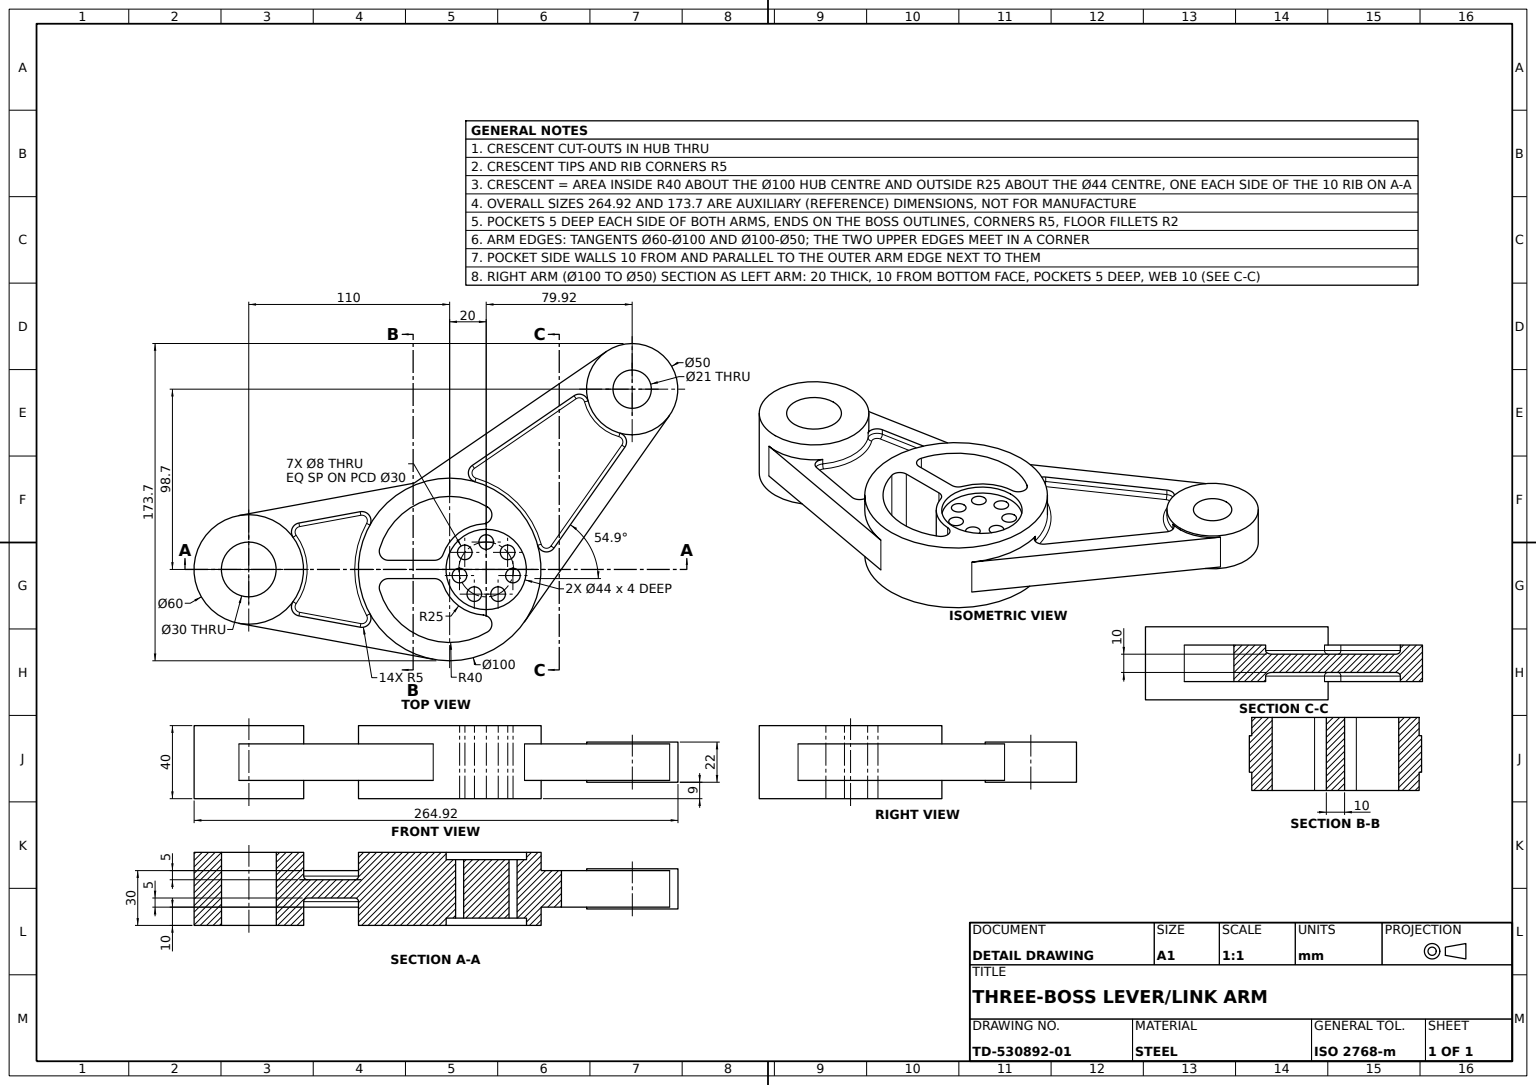
solid
v1 (-82.1770338609,5,-23.4495747344)
v2 (-82.5406702246,7,-25.4162390665)
e1 v1 v2 CIRCLE(AX(P(-82.1770338609,7,-23.4495747344),D(0.983332166,0,-0.1818181818),D(-0.1818181818,0,-0.983332166)),2)
v3 (-48.6283414749,5,-29.652730151)
e2 v3 v1 LINE
v4 (-48.9919778385,7,-31.619394483)
e3 v3 v4 CIRCLE(AX(P(-48.6283414749,7,-29.652730151),D(0.983332166,0,-0.1818181818),D(-0.1818181818,0,-0.983332166)),2)
e4 v2 v4 LINE
face CYL(AX(P(-6.9090909091,7,-37.3666223094),D(0.983332166,0,-0.1818181818),D(-0.1818181818,0,-0.983332166)),2) rev [-e1 -e2 e3 -e4]
v5 (57.1214748065,-7,-11.710555748)
v6 (57.1214748065,-10,-11.710555748)
e5 v5 v6 LINE
v7 (95.9321157128,-7,-66.9317168355)
e6 v5 v7 LINE
v8 (95.9321157128,-10,-66.9317168355)
e7 v7 v8 LINE
e8 v6 v8 LINE
face PLANE(AX(P(32.7258328837,10,23.0004317801),D(-0.8181458221,0,-0.5750107945),D(-0.5750107945,0,0.8181458221))) [-e5 e6 e7 -e8]
v9 (50.1381595672,-5,-13.7900310085)
v10 (14.4079942754,-5,-49.9640841101)
e9 v9 v10 CIRCLE(AX(P(0,-5,0),D(0,1,0),D(0,0,1)),52)
v11 (48.2097688146,-7,-13.2596452005)
e10 v9 v11 CIRCLE(AX(P(50.1381595672,-7,-13.7900310085),D(0.265192904,0,0.9641953763),D(0.9641953763,0,-0.265192904)),2)
v12 (13.8538406494,-7,-48.0423885674)
e11 v12 v11 CIRCLE(AX(P(0,-7,0),D(0,-1,0),D(0,0,1)),50)
e12 v10 v12 CIRCLE(AX(P(14.4079942754,-7,-49.9640841101),D(0.9608477713,0,0.277076813),D(0.277076813,0,-0.9608477713)),2)
face TORUS(AX(P(0,-7,0),D(0,1,0),D(0,0,1)),52,2) rev [-e9 e10 -e11 -e12]
v13 (-82.5406702246,10,-25.4162390665)
e13 v13 v2 LINE
v14 (-85.6842108418,10,-17.5710670597)
e14 v13 v14 CIRCLE(AX(P(-81.6315793155,10,-20.4995782363),D(0,1,0),D(0,0,1)),5)
v15 (-85.6842108418,7,-17.5710670597)
e15 v14 v15 LINE
e16 v15 v2 CIRCLE(AX(P(-81.6315793155,7,-20.4995782363),D(0,-1,0),D(0,0,1)),5)
face CYL(AX(P(-81.6315793155,10,-20.4995782363),D(0,-1,0),D(0,0,-1)),5) rev [-e13 e14 e15 e16]
v16 (-110,10,-30)
e17 v14 v16 CIRCLE(AX(P(-110,10,0),D(0,1,0),D(0,0,1)),30)
v17 (-110,20,-30)
e18 v17 v16 LINE
v18 (-110,20,30)
e19 v18 v17 CIRCLE(AX(P(-110,20,0),D(0,1,0),D(0,0,1)),30)
v19 (-110,10,30)
e20 v18 v19 LINE
v20 (-85.6842108418,10,17.5710670597)
e21 v19 v20 CIRCLE(AX(P(-110,10,0),D(0,1,0),D(0,0,1)),30)
v21 (-85.6842108418,7,17.5710670597)
e22 v20 v21 LINE
e23 v21 v15 CIRCLE(AX(P(-110,7,0),D(0,1,0),D(0,0,1)),30)
face CYL(AX(P(-110,20,0),D(0,-1,0),D(0,0,-1)),30) [e17 -e18 -e19 e20 e21 e22 e23 -e15]
v22 (5.3760813173,16,-0.6621859907)
v23 (5.3760813173,16,7.3378140093)
e24 v22 v23 CIRCLE(AX(P(5.3760813173,16,3.3378140093),D(0,1,0),D(0,0,1)),4)
v24 (5.3760813173,-16,7.3378140093)
e25 v23 v24 LINE
v25 (5.3760813173,-16,-0.6621859907)
e26 v25 v24 CIRCLE(AX(P(5.3760813173,-16,3.3378140093),D(0,1,0),D(0,0,1)),4)
e27 v22 v25 LINE
face CYL(AX(P(5.3760813173,16,3.3378140093),D(0,-1,0),D(0,0,-1)),4) rev [e24 e25 -e26 -e27]
v26 (20,-16,-19)
v27 (20,-16,-11)
e28 v26 v27 CIRCLE(AX(P(20,-16,-15),D(0,1,0),D(0,0,1)),4)
v28 (20,16,-19)
e29 v28 v26 LINE
v29 (20,16,-11)
e30 v28 v29 CIRCLE(AX(P(20,16,-15),D(0,1,0),D(0,0,1)),4)
e31 v29 v27 LINE
face CYL(AX(P(20,16,-15),D(0,-1,0),D(0,0,-1)),4) rev [-e28 -e29 e30 e31]
v30 (93.1884371125,10,-74.6218985242)
v31 (95.9321157128,10,-66.9317168355)
e32 v30 v31 CIRCLE(AX(P(91.8413866024,10,-69.806770808),D(0,-1,0),D(0,0,1)),5)
v32 (93.1884371125,7,-74.6218985242)
e33 v30 v32 LINE
v33 (95.9321157128,7,-66.9317168355)
e34 v32 v33 CIRCLE(AX(P(91.8413866024,7,-69.806770808),D(0,-1,0),D(0,0,1)),5)
e35 v31 v33 LINE
face CYL(AX(P(91.8413866024,10,-69.806770808),D(0,-1,0),D(0,0,-1)),5) rev [-e32 e33 e34 -e35]
v34 (-110,-20,15)
v35 (-110,-20,-15)
e36 v34 v35 CIRCLE(AX(P(-110,-20,0),D(0,1,0),D(0,0,1)),15)
v36 (-110,20,15)
e37 v36 v34 LINE
v37 (-110,20,-15)
e38 v36 v37 CIRCLE(AX(P(-110,20,0),D(0,1,0),D(0,0,1)),15)
e39 v37 v35 LINE
face CYL(AX(P(-110,20,0),D(0,-1,0),D(0,0,-1)),15) rev [-e36 -e37 e38 e39]
v38 (-110,-20,30)
v39 (-110,-20,-30)
e40 v38 v39 CIRCLE(AX(P(-110,-20,0),D(0,1,0),D(0,0,1)),30)
e41 v39 v38 CIRCLE(AX(P(-110,-20,0),D(0,1,0),D(0,0,1)),30)
e42 v35 v34 CIRCLE(AX(P(-110,-20,0),D(0,1,0),D(0,0,1)),15)
face PLANE(AX(P(-110,-20,0),D(0,1,0),D(0,0,1))) rev [-e40 -e41] [e36 e42]
v40 (69.2407418314,-5,-93.4480883396)
v41 (73.8341748162,-5,-91.7450400685)
e43 v40 v41 CIRCLE(AX(P(70.9353398332,-5,-90.9725403978),D(0,-1,0),D(0,0,1)),3)
v42 (68.1110098301,-7,-95.0984536341)
e44 v42 v40 CIRCLE(AX(P(69.2407418314,-7,-93.4480883396),D(0.8251826473,0,-0.5648660006),D(-0.5648660006,0,-0.8251826473)),2)
v43 (70.9353398332,-7,-95.9725403978)
e45 v43 v42 CIRCLE(AX(P(70.9353398332,-7,-90.9725403978),D(0,1,0),D(0,0,1)),5)
v44 (75.7667314716,-7,-92.260039849)
e46 v44 v43 CIRCLE(AX(P(70.9353398332,-7,-90.9725403978),D(0,1,0),D(0,0,1)),5)
e47 v44 v41 CIRCLE(AX(P(73.8341748162,-7,-91.7450400685),D(0.2574998902,0,0.9662783277),D(0.9662783277,0,-0.2574998902)),2)
face TORUS(AX(P(70.9353398332,-7,-90.9725403978),D(0,1,0),D(0,0,1)),3,2) rev [-e43 -e44 -e45 -e46 e47]
v45 (-38.3325939,-20,11.4285714286)
v46 (20.7142857143,-20,34.2186844772)
e48 v45 v46 CIRCLE(AX(P(0,-20,0),D(0,1,0),D(0,0,1)),40)
v47 (18.4375,-20,24.9511240979)
e49 v46 v47 CIRCLE(AX(P(18.125,-20,29.9413489175),D(0,1,0),D(0,0,-1)),5)
v48 (-3.5702260396,-20,8.3333333333)
e50 v47 v48 CIRCLE(AX(P(20,-20,0),D(0,-1,0),D(0,0,1)),25)
v49 (-8.2842712475,-20,5)
e51 v48 v49 CIRCLE(AX(P(-8.2842712475,-20,10),D(0,1,0),D(0,0,-1)),5)
v50 (-33.5410196625,-20,5)
e52 v49 v50 LINE
e53 v50 v45 CIRCLE(AX(P(-33.5410196625,-20,10),D(0,1,0),D(0,0,1)),5)
v51 (20,-20,22)
v52 (20,-20,-22)
e54 v51 v52 CIRCLE(AX(P(20,-20,0),D(0,1,0),D(0,0,1)),22)
e55 v52 v51 CIRCLE(AX(P(20,-20,0),D(0,1,0),D(0,0,1)),22)
v53 (20.7142857143,-20,-34.2186844772)
v54 (0,-20,-40)
e56 v53 v54 CIRCLE(AX(P(0,-20,0),D(0,1,0),D(0,0,1)),40)
v55 (-38.3325939,-20,-11.4285714286)
e57 v54 v55 CIRCLE(AX(P(0,-20,0),D(0,1,0),D(0,0,1)),40)
v56 (-33.5410196625,-20,-5)
e58 v55 v56 CIRCLE(AX(P(-33.5410196625,-20,-10),D(0,1,0),D(0,0,-1)),5)
v57 (-8.2842712475,-20,-5)
e59 v56 v57 LINE
v58 (-3.5702260396,-20,-8.3333333333)
e60 v57 v58 CIRCLE(AX(P(-8.2842712475,-20,-10),D(0,1,0),D(0,0,1)),5)
v59 (18.4375,-20,-24.9511240979)
e61 v58 v59 CIRCLE(AX(P(20,-20,0),D(0,-1,0),D(0,0,1)),25)
e62 v59 v53 CIRCLE(AX(P(18.125,-20,-29.9413489175),D(0,1,0),D(0,0,-1)),5)
v60 (0,-20,-50)
v61 (0,-20,50)
e63 v60 v61 CIRCLE(AX(P(0,-20,0),D(0,1,0),D(0,0,1)),50)
e64 v61 v60 CIRCLE(AX(P(0,-20,0),D(0,1,0),D(0,0,1)),50)
face PLANE(AX(P(0,-20,0),D(0,1,0),D(0,0,1))) rev [e48 e49 e50 e51 e52 e53] [e54 e55] [e56 e57 e58 e59 e60 e61 e62] [-e63 -e64]
v62 (50.1381595672,5,-13.7900310085)
v63 (53.0307456961,5,-11.5856097205)
e65 v62 v63 CIRCLE(AX(P(53.0307456961,5,-14.5856097205),D(0,1,0),D(0,0,1)),3)
v64 (55.4851831623,5,-12.860577337)
e66 v63 v64 CIRCLE(AX(P(53.0307456961,5,-14.5856097205),D(0,1,0),D(0,0,1)),3)
v65 (94.2958240686,5,-68.0817384245)
e67 v64 v65 LINE
v66 (92.6496169085,5,-72.6958474377)
e68 v65 v66 CIRCLE(AX(P(91.8413866024,5,-69.806770808),D(0,1,0),D(0,0,1)),3)
v67 (73.8341748162,5,-91.7450400685)
e69 v66 v67 CIRCLE(AX(P(99.9236896633,5,-98.697537105),D(0,-1,0),D(0,0,1)),27)
v68 (69.2407418314,5,-93.4480883396)
e70 v67 v68 CIRCLE(AX(P(70.9353398332,5,-90.9725403978),D(0,1,0),D(0,0,1)),3)
v69 (13.5446267125,5,-55.3221753659)
e71 v68 v69 LINE
v70 (14.4079942754,5,-49.9640841101)
e72 v69 v70 CIRCLE(AX(P(15.2392247144,5,-52.8466274241),D(0,1,0),D(0,0,1)),3)
e73 v70 v62 CIRCLE(AX(P(0,5,0),D(0,-1,0),D(0,0,1)),52)
face PLANE(AX(P(0,5,0),D(0,1,0),D(0,0,1))) [e65 e66 e67 e68 e69 e70 e71 e72 e73]
v71 (-82.5406702246,-7,-25.4162390665)
v72 (-85.6842108418,-7,-17.5710670597)
e74 v71 v72 CIRCLE(AX(P(-81.6315793155,-7,-20.4995782363),D(0,1,0),D(0,0,1)),5)
v73 (-85.6842108418,-10,-17.5710670597)
e75 v72 v73 LINE
v74 (-82.5406702246,-10,-25.4162390665)
e76 v74 v73 CIRCLE(AX(P(-81.6315793155,-10,-20.4995782363),D(0,1,0),D(0,0,1)),5)
e77 v71 v74 LINE
face CYL(AX(P(-81.6315793155,10,-20.4995782363),D(0,-1,0),D(0,0,-1)),5) rev [e74 e75 -e76 -e77]
v75 (-84.0631582313,5,18.7424715303)
e78 v21 v75 CIRCLE(AX(P(-84.0631582313,7,18.7424715303),D(-0.5857022353,0,0.8105263053),D(0.8105263053,0,0.5857022353)),2)
v76 (-84.0631582313,5,-18.7424715303)
e79 v76 v75 CIRCLE(AX(P(-110,5,0),D(0,-1,0),D(0,0,1)),32)
e80 v15 v76 CIRCLE(AX(P(-84.0631582313,7,-18.7424715303),D(0.5857022353,0,0.8105263053),D(0.8105263053,0,-0.5857022353)),2)
face TORUS(AX(P(-110,7,0),D(0,1,0),D(0,0,1)),32,2) rev [-e23 e78 -e79 -e80]
v77 (13.5446267125,-5,-55.3221753659)
e81 v10 v77 CIRCLE(AX(P(15.2392247144,-5,-52.8466274241),D(0,-1,0),D(0,0,1)),3)
v78 (12.4148947113,-7,-56.9725406605)
e82 v78 v12 CIRCLE(AX(P(15.2392247144,-7,-52.8466274241),D(0,1,0),D(0,0,1)),5)
e83 v78 v77 CIRCLE(AX(P(13.5446267125,-7,-55.3221753659),D(0.8251826473,0,-0.5648660006),D(-0.5648660006,0,-0.8251826473)),2)
face TORUS(AX(P(15.2392247144,-7,-52.8466274241),D(0,1,0),D(0,0,1)),3,2) rev [-e81 e12 -e82 e83]
v79 (20,16,22)
v80 (20,16,-22)
e84 v79 v80 CIRCLE(AX(P(20,16,0),D(0,1,0),D(0,0,1)),22)
v81 (20,20,22)
e85 v81 v79 LINE
v82 (20,20,-22)
e86 v81 v82 CIRCLE(AX(P(20,20,0),D(0,1,0),D(0,0,1)),22)
e87 v82 v80 LINE
face CYL(AX(P(20,20,0),D(0,-1,0),D(0,0,-1)),22) rev [-e84 -e85 e86 e87]
v83 (-48.0828869294,-7,-31.7027336528)
v84 (-48.9919778385,-7,-31.619394483)
e88 v83 v84 CIRCLE(AX(P(-48.0828869294,-7,-26.7027336528),D(0,1,0),D(0,0,1)),5)
v85 (-43.7117153904,-7,-24.2752124117)
e89 v85 v83 CIRCLE(AX(P(-48.0828869294,-7,-26.7027336528),D(0,1,0),D(0,0,1)),5)
v86 (-45.460184006,-5,-25.2462209081)
e90 v85 v86 CIRCLE(AX(P(-45.460184006,-7,-25.2462209081),D(-0.4855042482,0,0.8742343078),D(0.8742343078,0,0.4855042482)),2)
v87 (-48.6283414749,-5,-29.652730151)
e91 v87 v86 CIRCLE(AX(P(-48.0828869294,-5,-26.7027336528),D(0,-1,0),D(0,0,1)),3)
e92 v84 v87 CIRCLE(AX(P(-48.6283414749,-7,-29.652730151),D(0.983332166,0,-0.1818181818),D(-0.1818181818,0,-0.983332166)),2)
face TORUS(AX(P(-48.0828869294,-7,-26.7027336528),D(0,1,0),D(0,0,1)),3,2) rev [-e88 -e89 e90 -e91 -e92]
v88 (-48.9919778385,10,-31.619394483)
e93 v13 v88 LINE
v89 (-48.0828869294,10,-31.7027336528)
e94 v89 v88 CIRCLE(AX(P(-48.0828869294,10,-26.7027336528),D(0,1,0),D(0,0,1)),5)
v90 (-43.7117153904,10,-24.2752124117)
e95 v90 v89 CIRCLE(AX(P(-48.0828869294,10,-26.7027336528),D(0,1,0),D(0,0,1)),5)
v91 (0,10,-50)
e96 v91 v90 CIRCLE(AX(P(0,10,0),D(0,1,0),D(0,0,1)),50)
v92 (13.8538406494,10,-48.0423885674)
e97 v92 v91 CIRCLE(AX(P(0,10,0),D(0,1,0),D(0,0,1)),50)
v93 (12.4148947113,10,-56.9725406605)
e98 v92 v93 CIRCLE(AX(P(15.2392247144,10,-52.8466274241),D(0,-1,0),D(0,0,1)),5)
v94 (68.1110098301,10,-95.0984536341)
e99 v93 v94 LINE
v95 (70.9353398332,10,-95.9725403978)
e100 v95 v94 CIRCLE(AX(P(70.9353398332,10,-90.9725403978),D(0,1,0),D(0,0,1)),5)
v96 (75.7667314716,10,-92.260039849)
e101 v96 v95 CIRCLE(AX(P(70.9353398332,10,-90.9725403978),D(0,1,0),D(0,0,1)),5)
v97 (85.8020396479,10,-119.3271032867)
e102 v97 v96 CIRCLE(AX(P(99.9236896633,10,-98.697537105),D(0,1,0),D(0,0,1)),25)
v98 (-19.5045158411,10,-47.2411317325)
e103 v98 v97 LINE
v99 (-115.4545454545,10,-29.4999649811)
e104 v99 v98 LINE
e105 v16 v99 CIRCLE(AX(P(-110,10,0),D(0,1,0),D(0,0,1)),30)
face PLANE(AX(P(0,10,0),D(0,1,0),D(0,0,1))) [-e14 e93 -e94 -e95 -e96 -e97 e98 e99 -e100 -e101 -e102 -e103 -e104 -e105 -e17]
v100 (-48.9919778385,7,31.619394483)
v101 (-82.5406702246,7,25.4162390665)
e106 v100 v101 LINE
v102 (-48.6283414749,5,29.652730151)
e107 v100 v102 CIRCLE(AX(P(-48.6283414749,7,29.652730151),D(0.983332166,0,0.1818181818),D(0.1818181818,0,-0.983332166)),2)
v103 (-82.1770338609,5,23.4495747344)
e108 v103 v102 LINE
e109 v101 v103 CIRCLE(AX(P(-82.1770338609,7,23.4495747344),D(0.983332166,0,0.1818181818),D(0.1818181818,0,-0.983332166)),2)
face CYL(AX(P(-6.9090909091,7,37.3666223094),D(-0.983332166,0,-0.1818181818),D(-0.1818181818,0,0.983332166)),2) rev [-e106 e107 -e108 -e109]
v104 (68.1110098301,-10,-95.0984536341)
e110 v42 v104 LINE
e111 v42 v78 LINE
v105 (12.4148947113,-10,-56.9725406605)
e112 v78 v105 LINE
e113 v105 v104 LINE
face PLANE(AX(P(-22.5946400246,10,-33.0073058906),D(-0.5648660006,0,-0.8251826473),D(-0.8251826473,0,0.5648660006))) rev [-e110 e111 e112 e113]
e114 v88 v4 LINE
v106 (-48.0828869294,7,-31.7027336528)
e115 v4 v106 CIRCLE(AX(P(-48.0828869294,7,-26.7027336528),D(0,-1,0),D(0,0,1)),5)
e116 v89 v106 LINE
face CYL(AX(P(-48.0828869294,10,-26.7027336528),D(0,-1,0),D(0,0,-1)),5) rev [e94 e114 e115 -e116]
e117 v77 v40 LINE
face CYL(AX(P(-21.4649080234,-7,-31.3569405961),D(-0.8251826473,0,0.5648660006),D(0.5648660006,0,0.8251826473)),2) rev [-e83 -e111 e44 -e117]
v107 (20,-16,-22)
e118 v107 v52 LINE
v108 (20,-16,22)
e119 v107 v108 CIRCLE(AX(P(20,-16,0),D(0,1,0),D(0,0,1)),22)
e120 v108 v51 LINE
face CYL(AX(P(20,20,0),D(0,-1,0),D(0,0,-1)),22) rev [-e118 e119 e120 -e55]
v109 (57.1214748065,10,-11.710555748)
v110 (57.1214748065,7,-11.710555748)
e121 v109 v110 LINE
e122 v109 v31 LINE
e123 v33 v110 LINE
face PLANE(AX(P(32.7258328837,10,23.0004317801),D(-0.8181458221,0,-0.5750107945),D(-0.5750107945,0,0.8181458221))) [-e121 e122 e35 e123]
v111 (-48.9919778385,-7,31.619394483)
v112 (-48.9919778385,-10,31.619394483)
e124 v111 v112 LINE
v113 (-82.5406702246,-10,25.4162390665)
e125 v113 v112 LINE
v114 (-82.5406702246,-7,25.4162390665)
e126 v114 v113 LINE
e127 v114 v111 LINE
face PLANE(AX(P(-7.2727272727,10,39.3332866414),D(0.1818181818,0,-0.983332166),D(-0.983332166,0,-0.1818181818))) [e124 -e125 -e126 e127]
v115 (-82.5406702246,10,25.4162390665)
e128 v115 v101 LINE
e129 v101 v21 CIRCLE(AX(P(-81.6315793155,7,20.4995782363),D(0,-1,0),D(0,0,1)),5)
e130 v20 v115 CIRCLE(AX(P(-81.6315793155,10,20.4995782363),D(0,1,0),D(0,0,1)),5)
face CYL(AX(P(-81.6315793155,10,20.4995782363),D(0,-1,0),D(0,0,-1)),5) rev [e128 e129 -e22 e130]
v116 (-43.7117153904,-7,24.2752124117)
e131 v116 v85 CIRCLE(AX(P(0,-7,0),D(0,-1,0),D(0,0,1)),50)
v117 (-45.460184006,-5,25.2462209081)
e132 v116 v117 CIRCLE(AX(P(-45.460184006,-7,25.2462209081),D(0.4855042482,0,0.8742343078),D(0.8742343078,0,-0.4855042482)),2)
e133 v86 v117 CIRCLE(AX(P(0,-5,0),D(0,1,0),D(0,0,1)),52)
face TORUS(AX(P(0,-7,0),D(0,1,0),D(0,0,1)),52,2) rev [-e90 -e131 e132 -e133]
v118 (120.3773352156,10,-84.3222672425)
v119 (120.3773352156,-10,-84.3222672425)
e134 v118 v119 LINE
v120 (99.9236896633,-10,-73.697537105)
e135 v120 v119 CIRCLE(AX(P(99.9236896633,-10,-98.697537105),D(0,1,0),D(0,0,1)),25)
v121 (99.9236896633,-11,-73.697537105)
e136 v120 v121 LINE
v122 (99.9236896633,-11,-123.697537105)
e137 v121 v122 CIRCLE(AX(P(99.9236896633,-11,-98.697537105),D(0,1,0),D(0,0,1)),25)
v123 (99.9236896633,11,-123.697537105)
e138 v123 v122 LINE
v124 (99.9236896633,11,-73.697537105)
e139 v124 v123 CIRCLE(AX(P(99.9236896633,11,-98.697537105),D(0,1,0),D(0,0,1)),25)
v125 (99.9236896633,10,-73.697537105)
e140 v124 v125 LINE
e141 v125 v118 CIRCLE(AX(P(99.9236896633,10,-98.697537105),D(0,1,0),D(0,0,1)),25)
face CYL(AX(P(99.9236896633,11,-98.697537105),D(0,-1,0),D(0,0,-1)),25) [e134 -e135 e136 e137 -e138 -e139 e140 e141]
v126 (8.272527763,-16,-5.3523470279)
v127 (8.272527763,-16,-13.3523470279)
e142 v126 v127 CIRCLE(AX(P(8.272527763,-16,-9.3523470279),D(0,1,0),D(0,0,1)),4)
v128 (8.272527763,16,-5.3523470279)
e143 v128 v126 LINE
v129 (8.272527763,16,-13.3523470279)
e144 v128 v129 CIRCLE(AX(P(8.272527763,16,-9.3523470279),D(0,1,0),D(0,0,1)),4)
e145 v129 v127 LINE
face CYL(AX(P(8.272527763,16,-9.3523470279),D(0,-1,0),D(0,0,-1)),4) rev [-e142 -e143 e144 e145]
v130 (92.6496169085,-5,-72.6958474377)
e146 v41 v130 CIRCLE(AX(P(99.9236896633,-5,-98.697537105),D(0,1,0),D(0,0,1)),27)
v131 (93.1884371125,-7,-74.6218985242)
e147 v131 v44 CIRCLE(AX(P(99.9236896633,-7,-98.697537105),D(0,-1,0),D(0,0,1)),25)
e148 v131 v130 CIRCLE(AX(P(92.6496169085,-7,-72.6958474377),D(0.9630255432,0,0.269410102),D(0.269410102,0,-0.9630255432)),2)
face TORUS(AX(P(99.9236896633,-7,-98.697537105),D(0,1,0),D(0,0,1)),27,2) rev [-e146 -e47 -e147 e148]
v132 (75.7667314716,7,-92.260039849)
e149 v67 v132 CIRCLE(AX(P(73.8341748162,7,-91.7450400685),D(0.2574998902,0,0.9662783277),D(0.9662783277,0,-0.2574998902)),2)
v133 (70.9353398332,7,-95.9725403978)
e150 v133 v132 CIRCLE(AX(P(70.9353398332,7,-90.9725403978),D(0,-1,0),D(0,0,1)),5)
v134 (68.1110098301,7,-95.0984536341)
e151 v134 v133 CIRCLE(AX(P(70.9353398332,7,-90.9725403978),D(0,-1,0),D(0,0,1)),5)
e152 v68 v134 CIRCLE(AX(P(69.2407418314,7,-93.4480883396),D(0.8251826473,0,-0.5648660006),D(-0.5648660006,0,-0.8251826473)),2)
face TORUS(AX(P(70.9353398332,7,-90.9725403978),D(0,1,0),D(0,0,1)),3,2) rev [-e70 e149 -e150 -e151 -e152]
e153 v1 v76 CIRCLE(AX(P(-81.6315793155,5,-20.4995782363),D(0,1,0),D(0,0,1)),3)
face TORUS(AX(P(-81.6315793155,7,-20.4995782363),D(0,1,0),D(0,0,1)),3,2) rev [-e16 e80 -e153 e1]
v135 (-82.1770338609,-5,23.4495747344)
e154 v135 v114 CIRCLE(AX(P(-82.1770338609,-7,23.4495747344),D(0.983332166,0,0.1818181818),D(0.1818181818,0,-0.983332166)),2)
v136 (-85.6842108418,-7,17.5710670597)
e155 v136 v114 CIRCLE(AX(P(-81.6315793155,-7,20.4995782363),D(0,1,0),D(0,0,1)),5)
v137 (-84.0631582313,-5,18.7424715303)
e156 v137 v136 CIRCLE(AX(P(-84.0631582313,-7,18.7424715303),D(-0.5857022353,0,0.8105263053),D(0.8105263053,0,0.5857022353)),2)
e157 v135 v137 CIRCLE(AX(P(-81.6315793155,-5,20.4995782363),D(0,-1,0),D(0,0,1)),3)
face TORUS(AX(P(-81.6315793155,-7,20.4995782363),D(0,1,0),D(0,0,1)),3,2) rev [e154 -e155 -e156 -e157]
e158 v29 v28 CIRCLE(AX(P(20,16,-15),D(0,1,0),D(0,0,1)),4)
e159 v80 v79 CIRCLE(AX(P(20,16,0),D(0,1,0),D(0,0,1)),22)
v138 (31.727472237,16,-5.3523470279)
v139 (31.727472237,16,-13.3523470279)
e160 v138 v139 CIRCLE(AX(P(31.727472237,16,-9.3523470279),D(0,1,0),D(0,0,1)),4)
e161 v139 v138 CIRCLE(AX(P(31.727472237,16,-9.3523470279),D(0,1,0),D(0,0,1)),4)
v140 (26.5082560868,16,17.5145330185)
v141 (26.5082560868,16,9.5145330185)
e162 v140 v141 CIRCLE(AX(P(26.5082560868,16,13.5145330185),D(0,1,0),D(0,0,1)),4)
e163 v141 v140 CIRCLE(AX(P(26.5082560868,16,13.5145330185),D(0,1,0),D(0,0,1)),4)
v142 (13.4917439132,16,17.5145330185)
v143 (13.4917439132,16,9.5145330185)
e164 v142 v143 CIRCLE(AX(P(13.4917439132,16,13.5145330185),D(0,1,0),D(0,0,1)),4)
e165 v143 v142 CIRCLE(AX(P(13.4917439132,16,13.5145330185),D(0,1,0),D(0,0,1)),4)
v144 (34.6239186827,16,-0.6621859907)
v145 (34.6239186827,16,7.3378140093)
e166 v144 v145 CIRCLE(AX(P(34.6239186827,16,3.3378140093),D(0,1,0),D(0,0,1)),4)
e167 v145 v144 CIRCLE(AX(P(34.6239186827,16,3.3378140093),D(0,1,0),D(0,0,1)),4)
e168 v23 v22 CIRCLE(AX(P(5.3760813173,16,3.3378140093),D(0,1,0),D(0,0,1)),4)
e169 v129 v128 CIRCLE(AX(P(8.272527763,16,-9.3523470279),D(0,1,0),D(0,0,1)),4)
face PLANE(AX(P(20,16,0),D(0,1,0),D(0,0,1))) [-e30 -e158] [e159 e84] [-e160 -e161] [-e162 -e163] [-e164 -e165] [-e166 -e167] [-e24 -e168] [-e144 -e169]
v146 (-48.9919778385,-10,-31.619394483)
e170 v84 v146 LINE
v147 (-48.0828869294,-10,-31.7027336528)
e171 v147 v146 CIRCLE(AX(P(-48.0828869294,-10,-26.7027336528),D(0,1,0),D(0,0,1)),5)
e172 v83 v147 LINE
face CYL(AX(P(-48.0828869294,10,-26.7027336528),D(0,-1,0),D(0,0,-1)),5) rev [e170 -e171 -e172 e88]
v148 (-8.2842712475,20,5)
e173 v148 v49 LINE
v149 (-3.5702260396,20,8.3333333333)
e174 v149 v48 LINE
e175 v149 v148 CIRCLE(AX(P(-8.2842712475,20,10),D(0,1,0),D(0,0,-1)),5)
face CYL(AX(P(-8.2842712475,20,10),D(0,-1,0),D(0,0,-1)),5) rev [e173 -e51 -e174 e175]
v150 (-45.460184006,5,-25.2462209081)
v151 (-43.7117153904,7,-24.2752124117)
e176 v150 v151 CIRCLE(AX(P(-45.460184006,7,-25.2462209081),D(-0.4855042482,0,0.8742343078),D(0.8742343078,0,0.4855042482)),2)
e177 v106 v151 CIRCLE(AX(P(-48.0828869294,7,-26.7027336528),D(0,-1,0),D(0,0,1)),5)
e178 v150 v3 CIRCLE(AX(P(-48.0828869294,5,-26.7027336528),D(0,1,0),D(0,0,1)),3)
face TORUS(AX(P(-48.0828869294,7,-26.7027336528),D(0,1,0),D(0,0,1)),3,2) rev [e176 -e177 -e115 -e3 -e178]
v152 (13.8538406494,7,-48.0423885674)
v153 (12.4148947113,7,-56.9725406605)
e179 v152 v153 CIRCLE(AX(P(15.2392247144,7,-52.8466274241),D(0,-1,0),D(0,0,1)),5)
e180 v70 v152 CIRCLE(AX(P(14.4079942754,7,-49.9640841101),D(-0.9608477713,0,-0.277076813),D(-0.277076813,0,0.9608477713)),2)
e181 v69 v153 CIRCLE(AX(P(13.5446267125,7,-55.3221753659),D(0.8251826473,0,-0.5648660006),D(-0.5648660006,0,-0.8251826473)),2)
face TORUS(AX(P(15.2392247144,7,-52.8466274241),D(0,1,0),D(0,0,1)),3,2) rev [-e179 -e180 -e72 e181]
v154 (13.4917439132,-16,17.5145330185)
e182 v142 v154 LINE
v155 (13.4917439132,-16,9.5145330185)
e183 v143 v155 LINE
e184 v154 v155 CIRCLE(AX(P(13.4917439132,-16,13.5145330185),D(0,1,0),D(0,0,1)),4)
face CYL(AX(P(13.4917439132,16,13.5145330185),D(0,-1,0),D(0,0,-1)),4) rev [-e182 e164 e183 -e184]
v156 (93.1884371125,-10,-74.6218985242)
e185 v156 v8 CIRCLE(AX(P(91.8413866024,-10,-69.806770808),D(0,-1,0),D(0,0,1)),5)
e186 v7 v131 CIRCLE(AX(P(91.8413866024,-7,-69.806770808),D(0,1,0),D(0,0,1)),5)
e187 v131 v156 LINE
face CYL(AX(P(91.8413866024,10,-69.806770808),D(0,-1,0),D(0,0,-1)),5) rev [e185 -e7 e186 e187]
v157 (-48.6283414749,-5,29.652730151)
e188 v157 v111 CIRCLE(AX(P(-48.6283414749,-7,29.652730151),D(0.983332166,0,0.1818181818),D(0.1818181818,0,-0.983332166)),2)
v158 (-48.0828869294,-5,29.7027336528)
e189 v158 v157 CIRCLE(AX(P(-48.0828869294,-5,26.7027336528),D(0,-1,0),D(0,0,1)),3)
v159 (-48.0828869294,-7,31.7027336528)
e190 v159 v158 CIRCLE(AX(P(-48.0828869294,-7,29.7027336528),D(-1,0,0),D(0,0,1)),2)
e191 v111 v159 CIRCLE(AX(P(-48.0828869294,-7,26.7027336528),D(0,1,0),D(0,0,1)),5)
face TORUS(AX(P(-48.0828869294,-7,26.7027336528),D(0,1,0),D(0,0,1)),3,2) rev [-e188 -e189 -e190 -e191]
e192 v157 v135 LINE
face CYL(AX(P(-6.9090909091,-7,37.3666223094),D(0.983332166,0,0.1818181818),D(0.1818181818,0,-0.983332166)),2) rev [-e192 e188 -e127 -e154]
v160 (18.4375,20,24.9511240979)
e193 v160 v47 LINE
v161 (20.7142857143,20,34.2186844772)
e194 v161 v46 LINE
e195 v161 v160 CIRCLE(AX(P(18.125,20,29.9413489175),D(0,1,0),D(0,0,-1)),5)
face CYL(AX(P(18.125,20,29.9413489175),D(0,-1,0),D(0,0,-1)),5) rev [e193 -e49 -e194 e195]
v162 (-8.2842712475,20,-5)
e196 v162 v57 LINE
v163 (-3.5702260396,20,-8.3333333333)
e197 v162 v163 CIRCLE(AX(P(-8.2842712475,20,-10),D(0,1,0),D(0,0,1)),5)
e198 v163 v58 LINE
face CYL(AX(P(-8.2842712475,20,-10),D(0,-1,0),D(0,0,-1)),5) rev [-e196 e197 e198 -e60]
v164 (20.7142857143,20,-34.2186844772)
v165 (0,20,-40)
e199 v164 v165 CIRCLE(AX(P(0,20,0),D(0,1,0),D(0,0,1)),40)
e200 v165 v54 LINE
e201 v164 v53 LINE
face CYL(AX(P(0,20,0),D(0,-1,0),D(0,0,-1)),40) rev [e199 e200 -e56 -e201]
v166 (-48.9919778385,10,31.619394483)
e202 v166 v100 LINE
e203 v115 v166 LINE
face PLANE(AX(P(-7.2727272727,10,39.3332866414),D(0.1818181818,0,-0.983332166),D(-0.983332166,0,-0.1818181818))) [e202 e106 -e128 e203]
e204 v24 v25 CIRCLE(AX(P(5.3760813173,-16,3.3378140093),D(0,1,0),D(0,0,1)),4)
face CYL(AX(P(5.3760813173,16,3.3378140093),D(0,-1,0),D(0,0,-1)),4) rev [e168 e27 -e204 -e25]
e205 v93 v153 LINE
e206 v153 v134 LINE
e207 v94 v134 LINE
face PLANE(AX(P(-22.5946400246,10,-33.0073058906),D(-0.5648660006,0,-0.8251826473),D(-0.8251826473,0,0.5648660006))) rev [-e99 e205 e206 -e207]
e208 v96 v132 LINE
e209 v95 v133 LINE
face CYL(AX(P(70.9353398332,10,-90.9725403978),D(0,-1,0),D(0,0,-1)),5) rev [-e208 e101 e209 e150]
v167 (53.0307456961,7,-9.5856097205)
e210 v63 v167 CIRCLE(AX(P(53.0307456961,7,-11.5856097205),D(-1,0,0),D(0,0,1)),2)
v168 (48.2097688146,7,-13.2596452005)
e211 v168 v62 CIRCLE(AX(P(50.1381595672,7,-13.7900310085),D(0.265192904,0,0.9641953763),D(0.9641953763,0,-0.265192904)),2)
e212 v167 v168 CIRCLE(AX(P(53.0307456961,7,-14.5856097205),D(0,-1,0),D(0,0,1)),5)
face TORUS(AX(P(53.0307456961,7,-14.5856097205),D(0,1,0),D(0,0,1)),3,2) rev [-e210 -e65 -e211 -e212]
face PLANE(AX(P(-7.2727272727,10,-39.3332866414),D(-0.1818181818,0,-0.983332166),D(-0.983332166,0,0.1818181818))) rev [e13 e4 -e114 -e93]
v169 (-82.1770338609,-5,-23.4495747344)
e213 v169 v87 LINE
e214 v71 v169 CIRCLE(AX(P(-82.1770338609,-7,-23.4495747344),D(0.983332166,0,-0.1818181818),D(-0.1818181818,0,-0.983332166)),2)
e215 v84 v71 LINE
face CYL(AX(P(-6.9090909091,-7,-37.3666223094),D(-0.983332166,0,0.1818181818),D(0.1818181818,0,0.983332166)),2) rev [-e213 -e214 -e215 e92]
v170 (-43.7117153904,7,24.2752124117)
v171 (-48.0828869294,7,31.7027336528)
e216 v170 v171 CIRCLE(AX(P(-48.0828869294,7,26.7027336528),D(0,-1,0),D(0,0,1)),5)
v172 (-45.460184006,5,25.2462209081)
e217 v172 v170 CIRCLE(AX(P(-45.460184006,7,25.2462209081),D(0.4855042482,0,0.8742343078),D(0.8742343078,0,-0.4855042482)),2)
v173 (-48.0828869294,5,29.7027336528)
e218 v173 v172 CIRCLE(AX(P(-48.0828869294,5,26.7027336528),D(0,1,0),D(0,0,1)),3)
e219 v173 v171 CIRCLE(AX(P(-48.0828869294,7,29.7027336528),D(-1,0,0),D(0,0,1)),2)
face TORUS(AX(P(-48.0828869294,7,26.7027336528),D(0,1,0),D(0,0,1)),3,2) rev [-e216 -e217 -e218 e219]
v174 (13.8538406494,-10,-48.0423885674)
e220 v174 v105 CIRCLE(AX(P(15.2392247144,-10,-52.8466274241),D(0,-1,0),D(0,0,1)),5)
e221 v12 v174 LINE
face CYL(AX(P(15.2392247144,10,-52.8466274241),D(0,-1,0),D(0,0,-1)),5) rev [e220 -e112 e82 e221]
e222 v27 v26 CIRCLE(AX(P(20,-16,-15),D(0,1,0),D(0,0,1)),4)
face CYL(AX(P(20,16,-15),D(0,-1,0),D(0,0,-1)),4) rev [e158 e29 -e222 -e31]
v175 (-115.4545454545,10,29.4999649811)
v176 (-9.0909090909,10,49.1666083018)
e223 v175 v176 LINE
v177 (-43.7117153904,10,24.2752124117)
e224 v177 v176 CIRCLE(AX(P(0,10,0),D(0,1,0),D(0,0,1)),50)
e225 v166 v177 CIRCLE(AX(P(-48.0828869294,10,26.7027336528),D(0,1,0),D(0,0,1)),5)
e226 v175 v19 CIRCLE(AX(P(-110,10,0),D(0,1,0),D(0,0,1)),30)
face PLANE(AX(P(0,10,0),D(0,1,0),D(0,0,1))) [e223 -e224 -e225 -e203 -e130 -e21 -e226]
e227 v155 v154 CIRCLE(AX(P(13.4917439132,-16,13.5145330185),D(0,1,0),D(0,0,1)),4)
e228 v108 v107 CIRCLE(AX(P(20,-16,0),D(0,1,0),D(0,0,1)),22)
v178 (26.5082560868,-16,17.5145330185)
v179 (26.5082560868,-16,9.5145330185)
e229 v178 v179 CIRCLE(AX(P(26.5082560868,-16,13.5145330185),D(0,1,0),D(0,0,1)),4)
e230 v179 v178 CIRCLE(AX(P(26.5082560868,-16,13.5145330185),D(0,1,0),D(0,0,1)),4)
v180 (31.727472237,-16,-5.3523470279)
v181 (31.727472237,-16,-13.3523470279)
e231 v180 v181 CIRCLE(AX(P(31.727472237,-16,-9.3523470279),D(0,1,0),D(0,0,1)),4)
e232 v181 v180 CIRCLE(AX(P(31.727472237,-16,-9.3523470279),D(0,1,0),D(0,0,1)),4)
e233 v127 v126 CIRCLE(AX(P(8.272527763,-16,-9.3523470279),D(0,1,0),D(0,0,1)),4)
v182 (34.6239186827,-16,7.3378140093)
v183 (34.6239186827,-16,-0.6621859907)
e234 v182 v183 CIRCLE(AX(P(34.6239186827,-16,3.3378140093),D(0,1,0),D(0,0,1)),4)
e235 v183 v182 CIRCLE(AX(P(34.6239186827,-16,3.3378140093),D(0,1,0),D(0,0,1)),4)
face PLANE(AX(P(20,-16,0),D(0,1,0),D(0,0,1))) rev [e227 e184] [e204 e26] [-e119 -e228] [e28 e222] [e229 e230] [e231 e232] [e142 e233] [e234 e235]
v184 (-33.5410196625,20,5)
v185 (-38.3325939,20,11.4285714286)
e236 v184 v185 CIRCLE(AX(P(-33.5410196625,20,10),D(0,1,0),D(0,0,1)),5)
e237 v185 v45 LINE
e238 v184 v50 LINE
face CYL(AX(P(-33.5410196625,20,10),D(0,-1,0),D(0,0,-1)),5) rev [e236 e237 -e53 -e238]
v186 (18.4375,20,-24.9511240979)
e239 v186 v59 LINE
e240 v186 v164 CIRCLE(AX(P(18.125,20,-29.9413489175),D(0,1,0),D(0,0,-1)),5)
face CYL(AX(P(18.125,20,-29.9413489175),D(0,-1,0),D(0,0,-1)),5) rev [-e239 e240 e201 -e62]
v187 (53.0307456961,-5,-11.5856097205)
e241 v187 v9 CIRCLE(AX(P(53.0307456961,-5,-14.5856097205),D(0,-1,0),D(0,0,1)),3)
v188 (94.2958240686,-5,-68.0817384245)
e242 v130 v188 CIRCLE(AX(P(91.8413866024,-5,-69.806770808),D(0,-1,0),D(0,0,1)),3)
v189 (55.4851831623,-5,-12.860577337)
e243 v188 v189 LINE
e244 v189 v187 CIRCLE(AX(P(53.0307456961,-5,-14.5856097205),D(0,-1,0),D(0,0,1)),3)
face PLANE(AX(P(0,-5,0),D(0,1,0),D(0,0,1))) rev [e241 e9 e81 e117 e43 e146 e242 e243 e244]
face CYL(AX(P(20,20,0),D(0,-1,0),D(0,0,-1)),22) rev [e228 e118 -e54 -e120]
v190 (75.7667314716,-10,-92.260039849)
e245 v44 v190 LINE
v191 (85.8020396479,-10,-119.3271032867)
e246 v191 v190 CIRCLE(AX(P(99.9236896633,-10,-98.697537105),D(0,1,0),D(0,0,1)),25)
e247 v97 v191 LINE
e248 v132 v32 CIRCLE(AX(P(99.9236896633,7,-98.697537105),D(0,1,0),D(0,0,1)),25)
e249 v30 v125 CIRCLE(AX(P(99.9236896633,10,-98.697537105),D(0,1,0),D(0,0,1)),25)
e250 v123 v124 CIRCLE(AX(P(99.9236896633,11,-98.697537105),D(0,1,0),D(0,0,1)),25)
e251 v122 v121 CIRCLE(AX(P(99.9236896633,-11,-98.697537105),D(0,1,0),D(0,0,1)),25)
e252 v156 v120 CIRCLE(AX(P(99.9236896633,-10,-98.697537105),D(0,1,0),D(0,0,1)),25)
face CYL(AX(P(99.9236896633,11,-98.697537105),D(0,-1,0),D(0,0,-1)),25) [e147 e245 -e246 -e247 e102 e208 e248 -e33 e249 -e140 -e250 e138 e251 -e136 -e252 -e187]
e253 v171 v100 CIRCLE(AX(P(-48.0828869294,7,26.7027336528),D(0,-1,0),D(0,0,1)),5)
e254 v102 v173 CIRCLE(AX(P(-48.0828869294,5,26.7027336528),D(0,1,0),D(0,0,1)),3)
face TORUS(AX(P(-48.0828869294,7,26.7027336528),D(0,1,0),D(0,0,1)),3,2) rev [-e107 -e253 -e219 -e254]
v192 (48.2097688146,10,-13.2596452005)
e255 v109 v192 CIRCLE(AX(P(53.0307456961,10,-14.5856097205),D(0,-1,0),D(0,0,1)),5)
e256 v110 v167 CIRCLE(AX(P(53.0307456961,7,-14.5856097205),D(0,-1,0),D(0,0,1)),5)
e257 v192 v168 LINE
face CYL(AX(P(53.0307456961,10,-14.5856097205),D(0,-1,0),D(0,0,-1)),5) rev [-e255 e121 e256 e212 -e257]
v193 (99.9236896633,11,-109.197537105)
v194 (99.9236896633,11,-88.197537105)
e258 v193 v194 CIRCLE(AX(P(99.9236896633,11,-98.697537105),D(0,1,0),D(0,0,1)),10.5)
e259 v194 v193 CIRCLE(AX(P(99.9236896633,11,-98.697537105),D(0,1,0),D(0,0,1)),10.5)
face PLANE(AX(P(99.9236896633,11,-98.697537105),D(0,1,0),D(0,0,1))) [e250 e139] [-e258 -e259]
v195 (-115.4545454545,-10,-29.4999649811)
e260 v99 v195 LINE
v196 (-110,-10,-30)
e261 v196 v195 CIRCLE(AX(P(-110,-10,0),D(0,1,0),D(0,0,1)),30)
e262 v196 v39 LINE
v197 (-110,-10,30)
e263 v197 v38 LINE
v198 (-115.4545454545,-10,29.4999649811)
e264 v198 v197 CIRCLE(AX(P(-110,-10,0),D(0,1,0),D(0,0,1)),30)
e265 v175 v198 LINE
e266 v17 v18 CIRCLE(AX(P(-110,20,0),D(0,1,0),D(0,0,1)),30)
face CYL(AX(P(-110,20,0),D(0,-1,0),D(0,0,-1)),30) [e260 -e261 e262 e41 -e263 -e264 -e265 e226 -e20 -e266 e18 e105]
e267 v37 v36 CIRCLE(AX(P(-110,20,0),D(0,1,0),D(0,0,1)),15)
face PLANE(AX(P(-110,20,0),D(0,1,0),D(0,0,1))) [-e38 -e267] [e266 e19]
v199 (-38.3325939,20,-11.4285714286)
e268 v199 v55 LINE
v200 (-33.5410196625,20,-5)
e269 v199 v200 CIRCLE(AX(P(-33.5410196625,20,-10),D(0,1,0),D(0,0,-1)),5)
e270 v200 v56 LINE
face CYL(AX(P(-33.5410196625,20,-10),D(0,-1,0),D(0,0,-1)),5) rev [-e58 -e268 e269 e270]
v201 (40.9072911046,-10,28.7505397251)
e271 v201 v119 LINE
v202 (40.9072911046,10,28.7505397251)
e272 v202 v118 LINE
e273 v202 v201 LINE
face PLANE(AX(P(40.9072911046,10,28.7505397251),D(-0.8181458221,0,-0.5750107945),D(-0.5750107945,0,0.8181458221))) rev [e271 -e134 -e272 e273]
e274 v140 v178 LINE
e275 v141 v179 LINE
face CYL(AX(P(26.5082560868,16,13.5145330185),D(0,-1,0),D(0,0,-1)),4) rev [e163 e274 -e230 -e275]
e276 v72 v136 CIRCLE(AX(P(-110,-7,0),D(0,-1,0),D(0,0,1)),30)
v203 (-84.0631582313,-5,-18.7424715303)
e277 v203 v72 CIRCLE(AX(P(-84.0631582313,-7,-18.7424715303),D(0.5857022353,0,0.8105263053),D(0.8105263053,0,-0.5857022353)),2)
e278 v137 v203 CIRCLE(AX(P(-110,-5,0),D(0,1,0),D(0,0,1)),32)
face TORUS(AX(P(-110,-7,0),D(0,1,0),D(0,0,1)),32,2) rev [-e276 -e277 -e278 e156]
v204 (53.0307456961,-7,-9.5856097205)
e279 v204 v187 CIRCLE(AX(P(53.0307456961,-7,-11.5856097205),D(-1,0,0),D(0,0,1)),2)
e280 v11 v204 CIRCLE(AX(P(53.0307456961,-7,-14.5856097205),D(0,1,0),D(0,0,1)),5)
face TORUS(AX(P(53.0307456961,-7,-14.5856097205),D(0,1,0),D(0,0,1)),3,2) rev [-e10 -e241 -e279 -e280]
v205 (70.9353398332,-10,-95.9725403978)
e281 v43 v205 LINE
e282 v205 v104 CIRCLE(AX(P(70.9353398332,-10,-90.9725403978),D(0,1,0),D(0,0,1)),5)
face CYL(AX(P(70.9353398332,10,-90.9725403978),D(0,-1,0),D(0,0,-1)),5) rev [-e281 e45 e110 -e282]
e283 v139 v181 LINE
e284 v138 v180 LINE
face CYL(AX(P(31.727472237,16,-9.3523470279),D(0,-1,0),D(0,0,-1)),4) rev [e160 e283 -e231 -e284]
v206 (99.9236896633,-11,-109.197537105)
e285 v193 v206 LINE
v207 (99.9236896633,-11,-88.197537105)
e286 v207 v206 CIRCLE(AX(P(99.9236896633,-11,-98.697537105),D(0,1,0),D(0,0,1)),10.5)
e287 v194 v207 LINE
face CYL(AX(P(99.9236896633,11,-98.697537105),D(0,-1,0),D(0,0,-1)),10.5) rev [e259 e285 -e286 -e287]
e288 v82 v81 CIRCLE(AX(P(20,20,0),D(0,1,0),D(0,0,1)),22)
v208 (0,20,-50)
v209 (0,20,50)
e289 v208 v209 CIRCLE(AX(P(0,20,0),D(0,1,0),D(0,0,1)),50)
e290 v209 v208 CIRCLE(AX(P(0,20,0),D(0,1,0),D(0,0,1)),50)
e291 v165 v199 CIRCLE(AX(P(0,20,0),D(0,1,0),D(0,0,1)),40)
e292 v163 v186 CIRCLE(AX(P(20,20,0),D(0,-1,0),D(0,0,1)),25)
e293 v200 v162 LINE
e294 v185 v161 CIRCLE(AX(P(0,20,0),D(0,1,0),D(0,0,1)),40)
e295 v148 v184 LINE
e296 v160 v149 CIRCLE(AX(P(20,20,0),D(0,-1,0),D(0,0,1)),25)
face PLANE(AX(P(0,20,0),D(0,1,0),D(0,0,1))) [-e86 -e288] [e289 e290] [-e269 -e291 -e199 -e240 -e292 -e197 -e293] [-e195 -e294 -e236 -e295 -e175 -e296]
face CYL(AX(P(8.272527763,16,-9.3523470279),D(0,-1,0),D(0,0,-1)),4) rev [e143 -e233 -e145 e169]
face CYL(AX(P(0,20,0),D(0,-1,0),D(0,0,-1)),40) rev [e291 e268 -e57 -e200]
e297 v188 v7 CIRCLE(AX(P(94.2958240686,-7,-68.0817384245),D(0.5750107945,0,-0.8181458221),D(-0.8181458221,0,-0.5750107945)),2)
face TORUS(AX(P(91.8413866024,-7,-69.806770808),D(0,1,0),D(0,0,1)),3,2) rev [-e242 -e148 -e186 -e297]
v210 (-85.6842108418,-10,17.5710670597)
e298 v210 v113 CIRCLE(AX(P(-81.6315793155,-10,20.4995782363),D(0,1,0),D(0,0,1)),5)
e299 v136 v210 LINE
face CYL(AX(P(-81.6315793155,10,20.4995782363),D(0,-1,0),D(0,0,-1)),5) rev [e126 -e298 -e299 e155]
v211 (-43.7117153904,-10,24.2752124117)
e300 v112 v211 CIRCLE(AX(P(-48.0828869294,-10,26.7027336528),D(0,1,0),D(0,0,1)),5)
v212 (-9.0909090909,-10,49.1666083018)
e301 v211 v212 CIRCLE(AX(P(0,-10,0),D(0,1,0),D(0,0,1)),50)
e302 v198 v212 LINE
e303 v197 v210 CIRCLE(AX(P(-110,-10,0),D(0,1,0),D(0,0,1)),30)
face PLANE(AX(P(0,-10,0),D(0,1,0),D(0,0,1))) rev [e125 e300 e301 -e302 e264 e303 e298]
face CYL(AX(P(20,20,0),D(0,-1,0),D(0,0,-1)),22) rev [-e87 e288 e85 -e159]
face CYL(AX(P(-110,20,0),D(0,-1,0),D(0,0,-1)),15) rev [e37 -e42 -e39 e267]
face CYL(AX(P(20,20,0),D(0,-1,0),D(0,0,-1)),25) [-e193 e296 e174 -e50]
e304 v203 v169 CIRCLE(AX(P(-81.6315793155,-5,-20.4995782363),D(0,-1,0),D(0,0,1)),3)
e305 v117 v158 CIRCLE(AX(P(-48.0828869294,-5,26.7027336528),D(0,-1,0),D(0,0,1)),3)
face PLANE(AX(P(0,-5,0),D(0,1,0),D(0,0,1))) rev [e157 e278 e304 e213 e91 e133 e305 e189 e192]
face PLANE(AX(P(-8.2842712475,20,5),D(0,0,1),D(1,0,0))) [e238 -e52 -e173 e295]
e306 v144 v183 LINE
e307 v145 v182 LINE
face CYL(AX(P(34.6239186827,16,3.3378140093),D(0,-1,0),D(0,0,-1)),4) rev [-e306 e166 e307 -e235]
face CYL(AX(P(70.9353398332,10,-90.9725403978),D(0,-1,0),D(0,0,-1)),5) rev [e207 e151 -e209 e100]
v213 (-43.7117153904,-10,-24.2752124117)
e308 v213 v147 CIRCLE(AX(P(-48.0828869294,-10,-26.7027336528),D(0,1,0),D(0,0,1)),5)
e309 v85 v213 LINE
face CYL(AX(P(-48.0828869294,10,-26.7027336528),D(0,-1,0),D(0,0,-1)),5) rev [-e308 -e309 e89 e172]
e310 v189 v5 CIRCLE(AX(P(55.4851831623,-7,-12.860577337),D(0.5750107945,0,-0.8181458221),D(-0.8181458221,0,-0.5750107945)),2)
e311 v204 v5 CIRCLE(AX(P(53.0307456961,-7,-14.5856097205),D(0,1,0),D(0,0,1)),5)
face TORUS(AX(P(53.0307456961,-7,-14.5856097205),D(0,1,0),D(0,0,1)),3,2) rev [e279 -e244 e310 -e311]
e312 v151 v170 CIRCLE(AX(P(0,7,0),D(0,1,0),D(0,0,1)),50)
e313 v172 v150 CIRCLE(AX(P(0,5,0),D(0,-1,0),D(0,0,1)),52)
face TORUS(AX(P(0,7,0),D(0,1,0),D(0,0,1)),52,2) rev [e217 -e312 -e176 -e313]
e314 v176 v212 LINE
e315 v116 v211 LINE
v214 (0,-10,-50)
e316 v214 v213 CIRCLE(AX(P(0,-10,0),D(0,1,0),D(0,0,1)),50)
e317 v214 v60 LINE
e318 v209 v61 LINE
e319 v208 v91 LINE
e320 v90 v151 LINE
e321 v177 v170 LINE
face CYL(AX(P(0,20,0),D(0,-1,0),D(0,0,-1)),50) [e314 -e301 -e315 e131 e309 -e316 e317 e63 -e318 -e289 e319 e96 e320 e312 -e321 e224]
e322 v168 v152 CIRCLE(AX(P(0,7,0),D(0,1,0),D(0,0,1)),50)
face TORUS(AX(P(0,7,0),D(0,1,0),D(0,0,1)),52,2) rev [e180 -e322 e211 -e73]
e323 v75 v103 CIRCLE(AX(P(-81.6315793155,5,20.4995782363),D(0,1,0),D(0,0,1)),3)
face PLANE(AX(P(0,5,0),D(0,1,0),D(0,0,1))) [e108 e254 e218 e313 e178 e2 e153 e79 e323]
e324 v202 v192 CIRCLE(AX(P(0,10,0),D(0,1,0),D(0,0,1)),50)
face PLANE(AX(P(0,10,0),D(0,1,0),D(0,0,1))) [-e324 e272 -e141 -e249 e32 -e122 e255]
face CYL(AX(P(-48.0828869294,10,-26.7027336528),D(0,-1,0),D(0,0,-1)),5) rev [e116 e177 -e320 e95]
face CYL(AX(P(34.6239186827,16,3.3378140093),D(0,-1,0),D(0,0,-1)),4) rev [e306 -e234 -e307 e167]
e325 v110 v64 CIRCLE(AX(P(55.4851831623,7,-12.860577337),D(0.5750107945,0,-0.8181458221),D(-0.8181458221,0,-0.5750107945)),2)
face TORUS(AX(P(53.0307456961,7,-14.5856097205),D(0,1,0),D(0,0,1)),3,2) rev [e325 -e66 e210 -e256]
e326 v190 v205 CIRCLE(AX(P(70.9353398332,-10,-90.9725403978),D(0,1,0),D(0,0,1)),5)
face CYL(AX(P(70.9353398332,10,-90.9725403978),D(0,-1,0),D(0,0,-1)),5) rev [-e326 -e245 e46 e281]
v215 (48.2097688146,-10,-13.2596452005)
e327 v11 v215 LINE
e328 v201 v215 CIRCLE(AX(P(0,-10,0),D(0,1,0),D(0,0,1)),50)
e329 v92 v152 LINE
e330 v174 v214 CIRCLE(AX(P(0,-10,0),D(0,1,0),D(0,0,1)),50)
face CYL(AX(P(0,20,0),D(0,-1,0),D(0,0,-1)),50) [-e221 e11 e327 -e328 -e273 e324 e257 e322 -e329 e97 -e319 -e290 e318 e64 -e317 -e330]
face CYL(AX(P(-21.4649080234,7,-31.3569405961),D(0.8251826473,0,-0.5648660006),D(-0.5648660006,0,-0.8251826473)),2) rev [-e181 -e71 e152 -e206]
face CYL(AX(P(0,20,0),D(0,-1,0),D(0,0,-1)),40) rev [-e48 -e237 e294 e194]
e331 v33 v65 CIRCLE(AX(P(94.2958240686,7,-68.0817384245),D(0.5750107945,0,-0.8181458221),D(-0.8181458221,0,-0.5750107945)),2)
face CYL(AX(P(31.0895412395,7,21.8504101911),D(-0.5750107945,0,0.8181458221),D(0.8181458221,0,0.5750107945)),2) rev [-e325 -e123 e331 -e67]
v216 (-19.5045158411,-10,-47.2411317325)
e332 v195 v216 LINE
e333 v216 v191 LINE
e334 v74 v146 LINE
e335 v73 v196 CIRCLE(AX(P(-110,-10,0),D(0,1,0),D(0,0,1)),30)
face PLANE(AX(P(0,-10,0),D(0,1,0),D(0,0,1))) rev [e332 e333 e246 e326 e282 -e113 -e220 e330 e316 e308 e171 -e334 e76 e335 e261]
face PLANE(AX(P(-9.0909090909,10,49.1666083018),D(0.1818181818,0,-0.983332166),D(-0.983332166,0,-0.1818181818))) rev [e302 -e314 -e223 e265]
e336 v32 v66 CIRCLE(AX(P(92.6496169085,7,-72.6958474377),D(-0.9630255432,0,-0.269410102),D(-0.269410102,0,0.9630255432)),2)
face TORUS(AX(P(91.8413866024,7,-69.806770808),D(0,1,0),D(0,0,1)),3,2) rev [e336 -e68 -e331 -e34]
face TORUS(AX(P(-81.6315793155,7,20.4995782363),D(0,1,0),D(0,0,1)),3,2) rev [e109 -e323 -e78 -e129]
face CYL(AX(P(15.2392247144,10,-52.8466274241),D(0,-1,0),D(0,0,-1)),5) rev [-e98 e329 e179 -e205]
e337 v206 v207 CIRCLE(AX(P(99.9236896633,-11,-98.697537105),D(0,1,0),D(0,0,1)),10.5)
face PLANE(AX(P(99.9236896633,-11,-98.697537105),D(0,1,0),D(0,0,1))) rev [e286 e337] [-e137 -e251]
face CYL(AX(P(26.5082560868,16,13.5145330185),D(0,-1,0),D(0,0,-1)),4) rev [-e229 -e274 e162 e275]
e338 v98 v216 LINE
face PLANE(AX(P(-28.2433000308,10,-41.2591323633),D(-0.5648660006,0,-0.8251826473),D(-0.8251826473,0,0.5648660006))) [e103 e247 -e333 -e338]
face CYL(AX(P(31.727472237,16,-9.3523470279),D(0,-1,0),D(0,0,-1)),4) rev [-e232 -e283 e161 e284]
e339 v6 v215 CIRCLE(AX(P(53.0307456961,-10,-14.5856097205),D(0,-1,0),D(0,0,1)),5)
face PLANE(AX(P(0,-10,0),D(0,1,0),D(0,0,1))) rev [e328 -e339 e8 -e185 e252 e135 -e271]
e340 v159 v116 CIRCLE(AX(P(-48.0828869294,-7,26.7027336528),D(0,1,0),D(0,0,1)),5)
face TORUS(AX(P(-48.0828869294,-7,26.7027336528),D(0,1,0),D(0,0,1)),3,2) rev [-e132 -e340 e190 -e305]
face CYL(AX(P(31.0895412395,-7,21.8504101911),D(0.5750107945,0,-0.8181458221),D(-0.8181458221,0,-0.5750107945)),2) rev [-e243 e297 -e6 -e310]
face CYL(AX(P(13.4917439132,16,13.5145330185),D(0,-1,0),D(0,0,-1)),4) rev [e182 -e227 -e183 e165]
face CYL(AX(P(-48.0828869294,10,26.7027336528),D(0,-1,0),D(0,0,-1)),5) rev [-e124 e191 e340 e315 -e300]
face CYL(AX(P(-110,20,0),D(0,-1,0),D(0,0,-1)),30) [-e303 e263 e40 -e262 -e335 -e75 e276 e299]
face CYL(AX(P(53.0307456961,10,-14.5856097205),D(0,-1,0),D(0,0,-1)),5) rev [e339 -e327 e280 e311 e5]
face CYL(AX(P(99.9236896633,11,-98.697537105),D(0,-1,0),D(0,0,-1)),10.5) rev [e258 e287 -e337 -e285]
face TORUS(AX(P(99.9236896633,7,-98.697537105),D(0,1,0),D(0,0,1)),27,2) rev [-e336 -e248 -e149 -e69]
face CYL(AX(P(20,20,0),D(0,-1,0),D(0,0,-1)),25) [e292 e239 -e61 -e198]
face PLANE(AX(P(-8.2842712475,20,-5),D(0,0,-1),D(-1,0,0))) [e196 -e59 -e270 e293]
face TORUS(AX(P(-81.6315793155,-7,-20.4995782363),D(0,1,0),D(0,0,1)),3,2) rev [-e74 e214 -e304 e277]
face PLANE(AX(P(-9.0909090909,10,-49.1666083018),D(-0.1818181818,0,-0.983332166),D(-0.983332166,0,0.1818181818))) [e104 e338 -e332 -e260]
face CYL(AX(P(-48.0828869294,10,26.7027336528),D(0,-1,0),D(0,0,-1)),5) rev [e253 -e202 e225 e321 e216]
face PLANE(AX(P(-7.2727272727,10,-39.3332866414),D(-0.1818181818,0,-0.983332166),D(-0.983332166,0,0.1818181818))) rev [e334 -e170 e215 e77]
